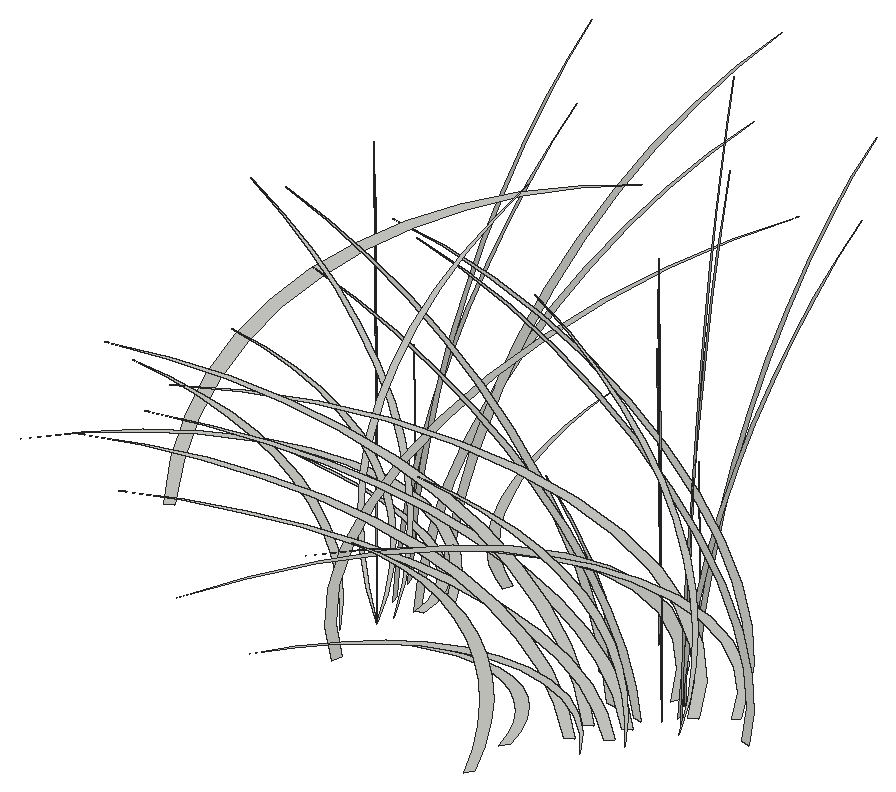
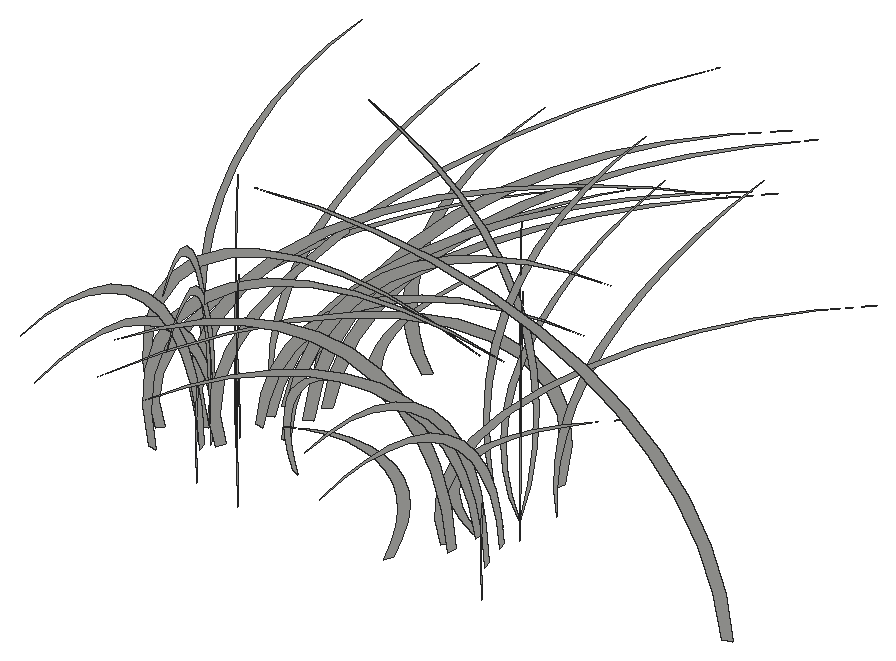
# SketchUp Ruby script. Lengths in inches.
U = 1.inch
M = Sketchup.active_model
def pt(a) = Geom::Point3d.new(a.map { |v| v * U })
def face(e, loops, mat)
  f = e.add_face(loops[0].map { |a| pt(a) })
  loops[1..].each { |l| e.add_face(l.map { |a| pt(a) }).erase! }
  f.material = f.back_material = mat if mat
  f
end
# faces: each face lists its corners as indices into pts; further lists are holes
def faces(e, pts, list, mat = nil) = list.each { |f| face(e, (f[0].is_a?(Array) ? f : [f]).map { |l| l.map { |i| pts[i] } }, mat) }
# xy, xz, yz: faces in a plane at the given z, y or x. An outline is a flat list of corners, or four numbers for a rectangle; further outlines are holes
def ring(l) = l.size == 4 ? [[l[0], l[1]], [l[2], l[1]], [l[2], l[3]], [l[0], l[3]]] : l.each_slice(2).to_a
def flat(e, list, mat, &to3) = list.each { |f| face(e, (f[0].is_a?(Array) ? f : [f]).map { |l| ring(l).map { |u, v| to3.(u, v) } }, mat) }
def xy(e, z, list, mat = nil) = flat(e, list, mat) { |x, y| [x, y, z] }
def xz(e, y, list, mat = nil) = flat(e, list, mat) { |x, z| [x, y, z] }
def yz(e, x, list, mat = nil) = flat(e, list, mat) { |y, z| [x, y, z] }
def lines(e, pts, list) = list.each { |a, b| e.add_line(pt(pts[a]), pt(pts[b])) }
# prism: a flat outline (further loops are holes) pulled along v
def prism(e, loops, v, mat = nil)
  f = face(e, loops, mat); d = Geom::Vector3d.new(v.map { |x| x * U })
  f.pushpull(f.normal.samedirection?(d) ? d.length : -d.length)
end
def box(e, o, s, mat = nil) = prism(e, [[o, [o[0] + s[0], o[1], o[2]], [o[0] + s[0], o[1] + s[1], o[2]], [o[0], o[1] + s[1], o[2]]]], [0, 0, s[2]], mat)
def at(x, y, z, deg = 0) = Geom::Transformation.translation(pt([x, y, z])) * Geom::Transformation.rotation(ORIGIN, Z_AXIS, deg.degrees)
def axes(o, x, y, z) = Geom::Transformation.new([*x, 0, *y, 0, *z, 0, *pt(o).to_a, 1])
def part(name) = M.definitions.add(name)
# library, detail: a bought-in or finely detailed component or shape, given as its bounding box
def library(name, o, s) = part(name).tap { |d| box(d.entities, o, s) }
def detail(e, o, s) = box(e.add_group.entities, o, s)
def put(e, d, t, mat = nil) = e.add_instance(d, t).tap { |i| i.material = mat if mat }
def group(e, t, mat = nil) = e.add_group.tap { |g| g.transformation = t; g.material = mat if mat }.entities
root = M.entities
g1 = group(root,at(387.49,274.53,0))
p = [[-0.5,-0.57,0],[-0.22,-0.25,0],[0,0,1.46],[-0.09,-0.1,2.93],[-0.49,-0.56,4.375],[-1.19,-1.35,5.75],
  [-2.17,-2.47,7.03],[-3.41,-3.89,8.18],[-4.88,-5.56,9.17],[-6.54,-7.45,9.98],[-8.36,-9.51,10.58],[-10.27,-11.69,10.97],
  [-12.24,-13.9375,11.125],[-14.23,-16.19,11.05],[-12.28,-13.98,11.0625],[-10.36,-11.79,10.86],[-8.5,-9.67,10.44],[-6.74,-7.67,9.82],
  [-5.13,-5.84,9.01],[-3.71,-4.22,8.02],[-2.51,-2.85,6.89],[-1.54,-1.76,5.64],[-0.85,-0.97,4.29],[-0.44,-0.5,2.88],
  [-0.32,-0.37,1.4375]]
faces(g1,p,[[0,1,2,3,4,5,6,7,8,9,10,11,12,13,14,15,16,17,18,19,20,21,22,23,24]])
g2 = group(root,at(384.38,274.21,0))
p = [[-6.07,19.87,18.05],[-6.99,22.87,18.53],[-6.1,19.96,17.95],[-5.25,17.16,17.15],[-4.43,14.49,16.14],[-3.66,11.97,14.93],
  [-2.95,9.65,13.53],[-2.31,7.54,11.96],[-1.73,5.67,10.23],[-1.24,4.06,8.37],[-0.83,2.72,6.39],[-0.51,1.68,4.32],
  [-0.29,0.94,2.18],[-0.16,0.52,0],[0,0,0],[-0.11,0.35,2.23],[-0.32,1.04,4.43],[-0.63,2.07,6.55],
  [-1.04,3.41,8.57],[-1.55,5.05,10.47],[-2.13,6.98,12.22],[-2.8,9.16,13.8],[-3.54,11.58,15.1875],[-4.34,14.1875,16.37],
  [-5.1875,16.96,17.33]]
faces(g2,p,[[0,1,2,3,4,5,6,7,8,9,10,11,12,13,14,15,16,17,18,19,20,21,22,23,24]])
g3 = group(root,at(383.32,276.15,0))
p = [[-4.56,5.55,7.88],[-3.72,4.53,7.38],[-2.97,3.62,6.83],[-2.31,2.81,6.24],[-1.73,2.11,5.62],[-1.26,1.54,4.96],
  [-0.89,1.09,4.27],[-0.63,0.76,3.57],[-0.47,0.58,2.86],[-0.43,0.52,2.13],[-0.49,0.6,1.41],[-0.67,0.81,0.7],
  [-0.95,1.16,0],[-0.59,0.71,0],[-0.27,0.33,0.71],[-0.07,0.09,1.43],[0,0,2.17],[-0.05,0.0625,2.9],
  [-0.22,0.27,3.63],[-0.52,0.63,4.34],[-0.93,1.13,5.03],[-1.45,1.77,5.69],[-2.09,2.54,6.3125],[-2.82,3.43,6.89],
  [-3.65,4.44,7.41]]
faces(g3,p,[[0,1,2,3,4,5,6,7,8,9,10,11,12,13,14,15,16,17,18,19,20,21,22,23,24]])
g4 = group(root,at(384.6,271.54,0))
p = [[-6.74,8.21,19.61],[-5.67,6.9,18.16],[-4.68,5.7,16.67],[-3.78,4.6,15.125],[-2.98,3.62,13.55],[-2.27,2.76,11.93],
  [-1.65,2.01,10.28],[-1.14,1.39,8.61],[-0.72,0.88,6.91],[-0.41,0.5,5.2],[-0.2,0.24,3.47],[-0.09,0.11,1.74],
  [-0.09,0.11,0],[0,0,1.74],[-0.03,0.04,3.49],[-0.1875,0.23,5.23],[-0.46,0.56,6.96],[-0.85,1.04,8.67],
  [-1.36,1.66,10.36],[-1.98,2.42,12.01],[-2.72,3.3125,13.63],[-3.57,4.35,15.21],[-4.52,5.51,16.73],[-5.58,6.8,18.2]]
faces(g4,p,[[0,1,2,3,4,5,6,7,8,9,10,11,12,13,14,15,16,17,18,19,20,21,22,23]])
g5 = group(root,at(384.6,271.54,0))
p = [[-6.74,8.21,19.61],[-5.67,6.9,18.16],[-4.68,5.7,16.67],[-3.78,4.6,15.125],[-2.98,3.62,13.55],[-2.27,2.76,11.93],
  [-1.65,2.01,10.28],[-1.14,1.39,8.61],[-0.72,0.88,6.91],[-0.41,0.5,5.2],[-0.2,0.24,3.47],[-0.09,0.11,1.74],
  [-0.09,0.11,0],[0,0,1.74],[-0.03,0.04,3.49],[-0.1875,0.23,5.23],[-0.46,0.56,6.96],[-0.85,1.04,8.67],
  [-1.36,1.66,10.36],[-1.98,2.42,12.01],[-2.72,3.3125,13.63],[-3.57,4.35,15.21],[-4.52,5.51,16.73],[-5.58,6.8,18.2]]
faces(g5,p,[[0,1,2,3,4,5,6,7,8,9,10,11,12,13,14,15,16,17,18,19,20,21,22,23]])
g6 = group(root,at(370.36,272.98,0.02))
p = [[19.18,7.98,20.75],[22.08,9.1875,21.3],[19.27,8.02,20.63],[16.57,6.9,19.72],[13.98,5.82,18.55],[11.56,4.8125,17.16],
  [9.32,3.88,15.55],[7.28,3.03,13.74],[5.47,2.28,11.76],[3.92,1.63,9.62],[2.63,1.09,7.35],[1.625,0.68,4.97],
  [0.91,0.38,2.51],[0.5,0.21,0],[0,0,0],[0.34,0.14,2.57],[1.01,0.42,5.09],[1.99,0.83,7.53],
  [3.29,1.37,9.85],[4.88,2.03,12.03],[6.74,2.81,14.04],[8.85,3.68,15.86],[11.18,4.65,17.46],[13.7,5.7,18.82],
  [16.375,6.82,19.92]]
faces(g6,p,[[0,1,2,3,4,5,6,7,8,9,10,11,12,13,14,15,16,17,18,19,20,21,22,23,24]])
g7 = group(root,at(384.94,272.36,0))
p = [[-6.07,19.87,14.56],[-6.99,22.87,14.94],[-6.1,19.96,14.48],[-5.25,17.16,13.83],[-4.43,14.49,13.02],[-3.66,11.97,12.04],
  [-2.95,9.65,10.91],[-2.31,7.54,9.64],[-1.73,5.67,8.25],[-1.24,4.06,6.75],[-0.83,2.72,5.15],[-0.51,1.68,3.49],
  [-0.29,0.94,1.76],[-0.16,0.52,0],[0,0,0],[-0.11,0.35,1.8],[-0.32,1.04,3.57],[-0.63,2.07,5.28],
  [-1.04,3.41,6.91],[-1.55,5.05,8.44],[-2.13,6.98,9.85],[-2.8,9.16,11.13],[-3.54,11.58,12.25],[-4.34,14.1875,13.2],
  [-5.1875,16.96,13.97]]
faces(g7,p,[[0,1,2,3,4,5,6,7,8,9,10,11,12,13,14,15,16,17,18,19,20,21,22,23,24]])
g8 = group(root,at(384.75,268.79,0))
p = [[-5.83,-8.875,16.67],[-4.9,-7.46,15.44],[-4.05,-6.16,14.17],[-3.27,-4.98,12.86],[-2.58,-3.92,11.51],[-1.96,-2.98,10.14],
  [-1.43,-2.18,8.74],[-0.99,-1.5,7.31],[-0.63,-0.95,5.87],[-0.36,-0.54,4.42],[-0.17,-0.26,2.95],[-0.08,-0.12,1.48],
  [-0.08,-0.12,0],[0,0,1.48],[-0.03,-0.04,2.97],[-0.16,-0.24,4.45],[-0.4,-0.6,5.92],[-0.74,-1.12,7.37],
  [-1.18,-1.79,8.81],[-1.72,-2.61,10.21],[-2.36,-3.58,11.59],[-3.09,-4.7,12.93],[-3.92,-5.96,14.22],[-4.83,-7.35,15.47]]
faces(g8,p,[[0,1,2,3,4,5,6,7,8,9,10,11,12,13,14,15,16,17,18,19,20,21,22,23]])
g9 = group(root,at(386.86,271.52,0))
p = [[-0.89,-0.32,0],[-0.4,-0.14,1.97],[-0.1,-0.04,3.96],[0,0,5.95],[-0.1,-0.03,7.95],[-0.39,-0.14,9.9375],
  [-0.89,-0.3125,11.91],[-1.57,-0.56,13.85],[-2.45,-0.87,15.76],[-3.52,-1.25,17.63],[-4.77,-1.6875,19.44],[-6.19,-2.19,21.2],
  [-7.79,-2.76,22.89],[-6.29,-2.23,21.17],[-4.94,-1.75,19.4],[-3.76,-1.33,17.58],[-2.74,-0.97,15.71],[-1.89,-0.67,13.8],
  [-1.22,-0.43,11.86],[-0.72,-0.25,9.9],[-0.4,-0.14,7.93],[-0.25,-0.09,5.94],[-0.29,-0.1,3.95],[-0.5,-0.18,1.97]]
faces(g9,p,[[0,1,2,3,4,5,6,7,8,9,10,11,12,13,14,15,16,17,18,19,20,21,22,23]])
g10 = group(root,at(387.96,272.875,0))
p = [[-9.01,-2.98,7.88],[-7.3,-2.41,7.38],[-5.75,-1.9,6.83],[-4.38,-1.45,6.24],[-3.2,-1.06,5.62],[-2.23,-0.74,4.96],
  [-1.47,-0.49,4.27],[-0.92,-0.31,3.57],[-0.61,-0.2,2.86],[-0.51,-0.17,2.13],[-0.65,-0.21,1.41],[-1.01,-0.33,0.7],
  [-1.6,-0.53,0],[-1.21,-0.4,0],[-0.54,-0.18,0.69],[-0.12,-0.04,1.4],[0.06,0.02,2.13],[-0.02,-0.01,2.85],
  [-0.35,-0.11,3.58],[-0.92,-0.3,4.29],[-1.73,-0.57,4.98],[-2.78,-0.92,5.64],[-4.05,-1.34,6.27],[-5.52,-1.82,6.86],
  [-7.18,-2.375,7.4]]
faces(g10,p,[[0,1,2,3,4,5,6,7,8,9,10,11,12,13,14,15,16,17,18,19,20,21,22,23,24]])
g11 = group(root,at(386.29,269.49,0))
p = [[-0.6,0.73,0],[-0.27,0.33,1.77],[-0.07,0.08,3.57],[0,0,5.36],[-0.07,0.08,7.16],[-0.27,0.32,8.95],
  [-0.6,0.73,10.73],[-1.06,1.29,12.48],[-1.65,2.01,14.2],[-2.37,2.88,15.88],[-3.21,3.91,17.52],[-4.17,5.08,19.1],
  [-5.25,6.39,20.625],[-4.23,5.15,19.08],[-3.33,4.05,17.48],[-2.53,3.08,15.83],[-1.84,2.25,14.15],[-1.27,1.55,12.43],
  [-0.82,1,10.6875],[-0.48,0.59,8.92],[-0.27,0.32,7.14],[-0.17,0.21,5.35],[-0.19,0.24,3.5625],[-0.34,0.41,1.78]]
faces(g11,p,[[0,1,2,3,4,5,6,7,8,9,10,11,12,13,14,15,16,17,18,19,20,21,22,23]])
g12 = group(root,at(386.21,271.01,0))
p = [[-0.52,-0.79,0],[-0.23,-0.35,1.51],[-0.06,-0.09,3.03],[0,0,4.56],[-0.06,-0.09,6.09],[-0.23,-0.35,7.61],
  [-0.52,-0.79,9.12],[-0.92,-1.39,10.61],[-1.43,-2.17,12.07],[-2.05,-3.12,13.5],[-2.78,-4.23,14.89],[-3.61,-5.49,16.24],
  [-4.54,-6.91,17.53],[-3.66,-5.57,16.21],[-2.88,-4.38,14.86],[-2.1875,-3.33,13.46],[-1.6,-2.43,12.03],[-1.1,-1.68,10.57],
  [-0.71,-1.08,9.08],[-0.42,-0.64,7.58],[-0.23,-0.35,6.07],[-0.15,-0.22,4.55],[-0.17,-0.25,3.03],[-0.29,-0.44,1.51]]
faces(g12,p,[[0,1,2,3,4,5,6,7,8,9,10,11,12,13,14,15,16,17,18,19,20,21,22,23]])
g13 = group(root,at(386.3125,272.24,0))
p = [[1.63,20.71,16.73],[1.875,23.84,17.17],[1.64,20.8125,16.64],[1.41,17.89,15.9],[1.1875,15.1,14.96],[0.98,12.48,13.84],
  [0.79,10.06,12.54],[0.62,7.86,11.08],[0.47,5.91,9.48],[0.33,4.23,7.76],[0.22,2.84,5.92],[0.14,1.75,4.01],
  [0.08,0.98,2.02],[0.04,0.54,0],[0,0,0],[0.03,0.36,2.07],[0.09,1.09,4.1],[0.17,2.15,6.07],
  [0.28,3.55,7.94],[0.41,5.27,9.7],[0.57,7.28,11.33],[0.75,9.55,12.79],[0.95,12.07,14.08],[1.16,14.79,15.17],
  [1.39,17.68,16.0625]]
faces(g13,p,[[0,1,2,3,4,5,6,7,8,9,10,11,12,13,14,15,16,17,18,19,20,21,22,23,24]])
g14 = group(root,at(386.47,274.17,0))
p = [[1.63,20.71,20.75],[1.875,23.84,21.3],[1.64,20.8125,20.63],[1.41,17.89,19.72],[1.1875,15.1,18.55],[0.98,12.48,17.16],
  [0.79,10.06,15.55],[0.62,7.86,13.74],[0.47,5.91,11.76],[0.33,4.23,9.62],[0.22,2.84,7.35],[0.14,1.75,4.97],
  [0.08,0.98,2.51],[0.04,0.54,0],[0,0,0],[0.03,0.36,2.57],[0.09,1.09,5.09],[0.17,2.15,7.53],
  [0.28,3.55,9.85],[0.41,5.27,12.03],[0.57,7.28,14.04],[0.75,9.55,15.86],[0.95,12.07,17.46],[1.16,14.79,18.82],
  [1.39,17.68,19.92]]
faces(g14,p,[[0,1,2,3,4,5,6,7,8,9,10,11,12,13,14,15,16,17,18,19,20,21,22,23,24]])
g15 = group(root,at(399.7,270.96,0))
p = [[-20.46,3.64,18.05],[-23.54,4.19,18.53],[-20.55,3.66,17.95],[-17.67,3.15,17.15],[-14.91,2.66,16.14],[-12.33,2.2,14.93],
  [-9.93,1.77,13.53],[-7.76,1.38,11.96],[-5.84,1.04,10.23],[-4.18,0.74,8.37],[-2.8,0.5,6.39],[-1.73,0.31,4.32],
  [-0.97,0.17,2.18],[-0.53,0.09,0],[0,0,0],[-0.36,0.0625,2.23],[-1.07,0.19,4.43],[-2.125,0.38,6.55],
  [-3.51,0.625,8.57],[-5.2,0.93,10.47],[-7.1875,1.28,12.22],[-9.43,1.68,13.8],[-11.92,2.125,15.1875],[-14.61,2.6,16.37],
  [-17.46,3.11,17.33]]
faces(g15,p,[[0,1,2,3,4,5,6,7,8,9,10,11,12,13,14,15,16,17,18,19,20,21,22,23,24]])
g16 = group(root,at(385.02,269.55,0))
p = [[0.67,0.67,0],[0.3,0.3,2.04],[0.08,0.08,4.1],[0,0,6.17],[0.07,0.07,8.23],[0.3,0.3,10.29],
  [0.66,0.66,12.33],[1.18,1.18,14.34],[1.84,1.84,16.32],[2.64,2.64,18.26],[3.58,3.58,20.14],[4.65,4.65,21.96],
  [5.84,5.84,23.71],[4.72,4.72,21.93],[3.71,3.71,20.09],[2.82,2.82,18.2],[2.05,2.05,16.26],[1.42,1.42,14.29],
  [0.91,0.91,12.29],[0.54,0.54,10.26],[0.3,0.3,8.21],[0.1875,0.1875,6.15],[0.22,0.22,4.09],[0.375,0.375,2.04]]
faces(g16,p,[[0,1,2,3,4,5,6,7,8,9,10,11,12,13,14,15,16,17,18,19,20,21,22,23]])
g17 = group(root,at(388.01,275.77,0))
p = [[2.34,6.79,9.0625],[1.91,5.55,8.49],[1.52,4.43,7.85],[1.18,3.44,7.18],[0.89,2.58,6.45],[0.65,1.88,5.7],
  [0.46,1.33,4.91],[0.32,0.93,4.1],[0.24,0.7,3.28],[0.22,0.64,2.45],[0.25,0.74,1.625],[0.34,1,0.8],
  [0.49,1.42,0],[0.3,0.875,0],[0.14,0.4,0.81],[0.04,0.11,1.65],[0,0,2.49],[0.03,0.07,3.34],
  [0.11,0.33,4.17],[0.27,0.77,4.99],[0.48,1.38,5.79],[0.75,2.17,6.54],[1.07,3.11,7.26],[1.45,4.2,7.92],
  [1.87,5.43,8.52]]
faces(g17,p,[[0,1,2,3,4,5,6,7,8,9,10,11,12,13,14,15,16,17,18,19,20,21,22,23,24]])
g18 = group(root,at(400.09,268.86,0))
p = [[-18.45,-9.5625,18.05],[-21.23,-11,18.53],[-18.53,-9.61,17.95],[-15.93,-8.26,17.15],[-13.45,-6.97,16.14],[-11.12,-5.76,14.93],
  [-8.96,-4.64,13.53],[-7,-3.63,11.96],[-5.26,-2.73,10.23],[-3.77,-1.95,8.37],[-2.53,-1.3125,6.39],[-1.5625,-0.81,4.32],
  [-0.875,-0.45,2.18],[-0.48,-0.25,0],[0,0,0],[-0.32,-0.17,2.23],[-0.97,-0.5,4.43],[-1.92,-0.99,6.55],
  [-3.16,-1.64,8.57],[-4.69,-2.43,10.47],[-6.48,-3.36,12.22],[-8.51,-4.41,13.8],[-10.75,-5.57,15.1875],[-13.17,-6.83,16.37],
  [-15.75,-8.16,17.33]]
faces(g18,p,[[0,1,2,3,4,5,6,7,8,9,10,11,12,13,14,15,16,17,18,19,20,21,22,23,24]])
g19 = group(root,at(400.09,268.86,0))
p = [[-18.45,-9.5625,18.05],[-21.23,-11,18.53],[-18.53,-9.61,17.95],[-15.93,-8.26,17.15],[-13.45,-6.97,16.14],[-11.12,-5.76,14.93],
  [-8.96,-4.64,13.53],[-7,-3.63,11.96],[-5.26,-2.73,10.23],[-3.77,-1.95,8.37],[-2.53,-1.3125,6.39],[-1.5625,-0.81,4.32],
  [-0.875,-0.45,2.18],[-0.48,-0.25,0],[0,0,0],[-0.32,-0.17,2.23],[-0.97,-0.5,4.43],[-1.92,-0.99,6.55],
  [-3.16,-1.64,8.57],[-4.69,-2.43,10.47],[-6.48,-3.36,12.22],[-8.51,-4.41,13.8],[-10.75,-5.57,15.1875],[-13.17,-6.83,16.37],
  [-15.75,-8.16,17.33]]
faces(g19,p,[[0,1,2,3,4,5,6,7,8,9,10,11,12,13,14,15,16,17,18,19,20,21,22,23,24]])
g20 = group(root,at(401.6,270.62,0))
p = [[-20.46,3.64,14.56],[-23.54,4.19,14.94],[-20.55,3.66,14.48],[-17.67,3.15,13.83],[-14.91,2.66,13.02],[-12.33,2.2,12.04],
  [-9.93,1.77,10.91],[-7.76,1.38,9.64],[-5.84,1.04,8.25],[-4.18,0.74,6.75],[-2.8,0.5,5.15],[-1.73,0.31,3.49],
  [-0.97,0.17,1.76],[-0.53,0.09,0],[0,0,0],[-0.36,0.0625,1.8],[-1.07,0.19,3.57],[-2.125,0.38,5.28],
  [-3.51,0.625,6.91],[-5.2,0.93,8.44],[-7.1875,1.28,9.85],[-9.43,1.68,11.13],[-11.92,2.125,12.25],[-14.61,2.6,13.2],
  [-17.46,3.11,13.97]]
faces(g20,p,[[0,1,2,3,4,5,6,7,8,9,10,11,12,13,14,15,16,17,18,19,20,21,22,23,24]])
g21 = group(root,at(386.16,265.61,0))
p = [[0.26,0.96,0],[0.11,0.43,0],[0,0,2.01],[0.05,0.17,4.04],[0.25,0.9375,6.02],[0.62,2.28,7.92],
  [1.125,4.16,9.68],[1.76,6.54,11.26],[2.52,9.35,12.62],[3.38,12.53,13.73],[4.32,16,14.5625],[5.31,19.67,15.09],
  [6.33,23.45,15.31],[7.35,27.24,15.2],[6.35,23.52,15.22],[5.35,19.83,14.94],[4.39,16.27,14.37],[3.48,12.91,13.51],
  [2.65,9.83,12.39],[1.92,7.11,11.04],[1.29,4.8,9.48],[0.8,2.96,7.75],[0.44,1.63,5.9],[0.23,0.84,3.96],
  [0.17,0.62,1.98]]
faces(g21,p,[[0,1,2,3,4,5,6,7,8,9,10,11,12,13,14,15,16,17,18,19,20,21,22,23,24]])
g22 = group(root,at(400.14,267.37,0))
p = [[-17.17,-11.7,15.34],[-19.76,-13.47,15.75],[-17.25,-11.76,15.26],[-14.83,-10.11,14.58],[-12.52,-8.53,13.72],[-10.35,-7.05,12.69],
  [-8.34,-5.68,11.5],[-6.52,-4.44,10.16],[-4.9,-3.34,8.7],[-3.51,-2.39,7.11],[-2.35,-1.6,5.43],[-1.45,-0.99,3.67],
  [-0.82,-0.56,1.86],[-0.45,-0.3,0],[0,0,0],[-0.3,-0.21,1.9],[-0.9,-0.61,3.76],[-1.78,-1.22,5.57],
  [-2.95,-2.01,7.28],[-4.37,-2.98,8.9],[-6.03,-4.11,10.39],[-7.92,-5.4,11.73],[-10,-6.82,12.91],[-12.26,-8.36,13.91],
  [-14.66,-9.99,14.73]]
faces(g22,p,[[0,1,2,3,4,5,6,7,8,9,10,11,12,13,14,15,16,17,18,19,20,21,22,23,24]])
g23 = group(root,at(401.81,269.75,0))
p = [[-18.45,-9.5625,14.56],[-21.23,-11,14.94],[-18.53,-9.61,14.48],[-15.93,-8.26,13.83],[-13.45,-6.97,13.02],[-11.12,-5.76,12.04],
  [-8.96,-4.64,10.91],[-7,-3.63,9.64],[-5.26,-2.73,8.25],[-3.77,-1.95,6.75],[-2.53,-1.3125,5.15],[-1.5625,-0.81,3.49],
  [-0.875,-0.45,1.76],[-0.48,-0.25,0],[0,0,0],[-0.32,-0.17,1.8],[-0.97,-0.5,3.57],[-1.92,-0.99,5.28],
  [-3.16,-1.64,6.91],[-4.69,-2.43,8.44],[-6.48,-3.36,9.85],[-8.51,-4.41,11.13],[-10.75,-5.57,12.25],[-13.17,-6.83,13.2],
  [-15.75,-8.16,13.97]]
faces(g23,p,[[0,1,2,3,4,5,6,7,8,9,10,11,12,13,14,15,16,17,18,19,20,21,22,23,24]])
g24 = group(root,at(401.81,269.75,0))
p = [[-18.45,-9.5625,14.56],[-21.23,-11,14.94],[-18.53,-9.61,14.48],[-15.93,-8.26,13.83],[-13.45,-6.97,13.02],[-11.12,-5.76,12.04],
  [-8.96,-4.64,10.91],[-7,-3.63,9.64],[-5.26,-2.73,8.25],[-3.77,-1.95,6.75],[-2.53,-1.3125,5.15],[-1.5625,-0.81,3.49],
  [-0.875,-0.45,1.76],[-0.48,-0.25,0],[0,0,0],[-0.32,-0.17,1.8],[-0.97,-0.5,3.57],[-1.92,-0.99,5.28],
  [-3.16,-1.64,6.91],[-4.69,-2.43,8.44],[-6.48,-3.36,9.85],[-8.51,-4.41,11.13],[-10.75,-5.57,12.25],[-13.17,-6.83,13.2],
  [-15.75,-8.16,13.97]]
faces(g24,p,[[0,1,2,3,4,5,6,7,8,9,10,11,12,13,14,15,16,17,18,19,20,21,22,23,24]])
g25 = group(root,at(404.67,275.47,0))
p = [[-0.91,0.16,0],[-0.4,0.07,0],[0,0,2.0625],[-0.16,0.03,4.13],[-0.89,0.16,6.16],[-2.17,0.39,8.1],
  [-3.95,0.7,9.91],[-6.21,1.11,11.52],[-8.88,1.58,12.92],[-11.91,2.12,14.05],[-15.2,2.71,14.9],[-18.68,3.33,15.45],
  [-22.27,3.97,15.67],[-25.88,4.61,15.5625],[-22.34,3.98,15.58],[-18.84,3.36,15.29],[-15.45,2.75,14.71],[-12.26,2.18,13.83],
  [-9.34,1.66,12.68],[-6.75,1.2,11.3],[-4.56,0.8125,9.7],[-2.81,0.5,7.9375],[-1.55,0.28,6.04],[-0.8,0.14,4.05],
  [-0.59,0.1,2.02]]
faces(g25,p,[[0,1,2,3,4,5,6,7,8,9,10,11,12,13,14,15,16,17,18,19,20,21,22,23,24]])
g26 = group(root,at(404.67,275.47,0))
p = [[-0.91,0.16,0],[-0.4,0.07,0],[0,0,2.0625],[-0.16,0.03,4.13],[-0.89,0.16,6.16],[-2.17,0.39,8.1],
  [-3.95,0.7,9.91],[-6.21,1.11,11.52],[-8.88,1.58,12.92],[-11.91,2.12,14.05],[-15.2,2.71,14.9],[-18.68,3.33,15.45],
  [-22.27,3.97,15.67],[-25.88,4.61,15.5625],[-22.34,3.98,15.58],[-18.84,3.36,15.29],[-15.45,2.75,14.71],[-12.26,2.18,13.83],
  [-9.34,1.66,12.68],[-6.75,1.2,11.3],[-4.56,0.8125,9.7],[-2.81,0.5,7.9375],[-1.55,0.28,6.04],[-0.8,0.14,4.05],
  [-0.59,0.1,2.02]]
faces(g26,p,[[0,1,2,3,4,5,6,7,8,9,10,11,12,13,14,15,16,17,18,19,20,21,22,23,24]])
g27 = group(root,at(401.73,268.46,0))
p = [[-17.17,-11.7,12.375],[-19.76,-13.47,12.7],[-17.25,-11.76,12.31],[-14.83,-10.11,11.76],[-12.52,-8.53,11.07],[-10.35,-7.05,10.23],
  [-8.34,-5.68,9.27],[-6.52,-4.44,8.2],[-4.9,-3.34,7.01],[-3.51,-2.39,5.74],[-2.35,-1.6,4.38],[-1.45,-0.99,2.96],
  [-0.82,-0.56,1.5],[-0.45,-0.3,0],[0,0,0],[-0.3,-0.21,1.53],[-0.9,-0.61,3.03],[-1.78,-1.22,4.49],
  [-2.95,-2.01,5.875],[-4.37,-2.98,7.18],[-6.03,-4.11,8.375],[-7.92,-5.4,9.46],[-10,-6.82,10.41],[-12.26,-8.36,11.22],
  [-14.66,-9.99,11.88]]
faces(g27,p,[[0,1,2,3,4,5,6,7,8,9,10,11,12,13,14,15,16,17,18,19,20,21,22,23,24]])
g28 = group(root,at(403.93,272.77,0))
p = [[-0.82,-0.43,0],[-0.36,-0.1875,0],[0,0,2.0625],[-0.15,-0.08,4.13],[-0.8,-0.42,6.16],[-1.95,-1.01,8.1],
  [-3.57,-1.85,9.91],[-5.6,-2.9,11.52],[-8.01,-4.15,12.92],[-10.74,-5.57,14.05],[-13.71,-7.1,14.9],[-16.85,-8.73,15.45],
  [-20.09,-10.41,15.67],[-23.34,-12.1,15.5625],[-20.15,-10.44,15.58],[-16.99,-8.81,15.29],[-13.9375,-7.22,14.71],[-11.06,-5.73,13.83],
  [-8.42,-4.37,12.68],[-6.09,-3.16,11.3],[-4.11,-2.13,9.7],[-2.53,-1.3125,7.9375],[-1.4,-0.72,6.04],[-0.72,-0.375,4.05],
  [-0.53,-0.27,2.02]]
faces(g28,p,[[0,1,2,3,4,5,6,7,8,9,10,11,12,13,14,15,16,17,18,19,20,21,22,23,24]])
g29 = group(root,at(407.53,271.91,0))
p = [[-0.95,0.28,0],[-0.42,0.125,0],[0,0,2.01],[-0.17,0.05,4.04],[-0.93,0.27,6.02],[-2.27,0.66,7.92],
  [-4.14,1.21,9.68],[-6.5,1.9,11.26],[-9.3,2.72,12.62],[-12.46,3.64,13.73],[-15.91,4.65,14.5625],[-19.55,5.72,15.09],
  [-23.3125,6.82,15.31],[-27.08,7.92,15.2],[-23.38,6.84,15.22],[-19.72,5.77,14.94],[-16.17,4.73,14.37],[-12.83,3.75,13.51],
  [-9.77,2.86,12.39],[-7.0625,2.07,11.04],[-4.77,1.39,9.48],[-2.94,0.86,7.75],[-1.62,0.47,5.9],[-0.84,0.25,3.96],
  [-0.61,0.18,1.98]]
faces(g29,p,[[0,1,2,3,4,5,6,7,8,9,10,11,12,13,14,15,16,17,18,19,20,21,22,23,24]])
g30 = group(root,at(398.26,272.65,0))
p = [[-6.53,2.99,7.88],[-5.33,2.44,7.38],[-4.26,1.95,6.83],[-3.3,1.51,6.24],[-2.48,1.14,5.62],[-1.81,0.83,4.96],
  [-1.28,0.58,4.27],[-0.9,0.41,3.57],[-0.68,0.31,2.86],[-0.61,0.28,2.13],[-0.71,0.32,1.41],[-0.96,0.4375,0.7],
  [-1.37,0.625,0],[-0.84,0.38,0],[-0.39,0.18,0.71],[-0.11,0.05,1.43],[0,0,2.17],[-0.07,0.03,2.9],
  [-0.32,0.15,3.63],[-0.74,0.34,4.34],[-1.33,0.61,5.03],[-2.08,0.95,5.69],[-2.99,1.37,6.3125],[-4.04,1.85,6.89],
  [-5.22,2.39,7.41]]
faces(g30,p,[[0,1,2,3,4,5,6,7,8,9,10,11,12,13,14,15,16,17,18,19,20,21,22,23,24]])
g31 = group(root,at(401.02,272.88,0))
p = [[-10.66,12.98,9.9],[-9.23,11.23,9.83],[-7.82,9.52,9.59],[-6.46,7.86,9.18],[-5.18,6.3,8.61],[-3.99,4.86,7.88],
  [-2.93,3.57,7.02],[-2.02,2.46,6.03],[-1.27,1.54,4.95],[-0.6875,0.84,3.78],[-0.29,0.36,2.55],[-0.1,0.12,1.28],
  [-0.09,0.12,0],[0,0,1.3],[-0.125,0.15,2.61],[-0.47,0.57,3.875],[-1.02,1.24,5.09],[-1.77,2.15,6.21],
  [-2.69,3.28,7.22],[-3.78,4.6,8.1],[-5,6.09,8.82],[-6.33,7.71,9.37],[-7.74,9.43,9.74],[-9.2,11.19,9.92]]
faces(g31,p,[[0,1,2,3,4,5,6,7,8,9,10,11,12,13,14,15,16,17,18,19,20,21,22,23]])
g32 = group(root,at(402.28,273.16,0))
p = [[-11.32,17.43,20.75],[-13.02,20.05,21.3],[-11.37,17.51,20.63],[-9.77,15.05,19.72],[-8.25,12.7,18.55],[-6.82,10.5,17.16],
  [-5.5,8.46,15.55],[-4.29,6.61,13.74],[-3.23,4.97,11.76],[-2.3125,3.56,9.62],[-1.55,2.39,7.35],[-0.96,1.47,4.97],
  [-0.54,0.83,2.51],[-0.29,0.45,0],[0,0,0],[-0.2,0.31,2.57],[-0.59,0.91,5.09],[-1.18,1.8125,7.53],
  [-1.94,2.99,9.85],[-2.88,4.43,12.03],[-3.98,6.12,14.04],[-5.22,8.04,15.86],[-6.59,10.15,17.46],[-8.08,12.44,18.82],
  [-9.66,14.88,19.92]]
faces(g32,p,[[0,1,2,3,4,5,6,7,8,9,10,11,12,13,14,15,16,17,18,19,20,21,22,23,24]])
g33 = group(root,at(398.15,276.375,0))
p = [[-4.56,5.55,16.02],[-3.72,4.53,15.01],[-2.97,3.62,13.89],[-2.31,2.81,12.69],[-1.73,2.11,11.42],[-1.26,1.54,10.08],
  [-0.89,1.09,8.6875],[-0.63,0.76,7.26],[-0.47,0.58,5.8],[-0.43,0.52,4.34],[-0.49,0.6,2.87],[-0.67,0.81,1.42],
  [-0.95,1.16,0],[-0.59,0.71,0],[-0.27,0.33,1.44],[-0.07,0.09,2.92],[0,0,4.41],[-0.05,0.0625,5.9],
  [-0.22,0.27,7.38],[-0.52,0.63,8.83],[-0.93,1.13,10.23],[-1.45,1.77,11.57],[-2.09,2.54,12.83],[-2.82,3.43,14.01],
  [-3.65,4.44,15.07]]
faces(g33,p,[[0,1,2,3,4,5,6,7,8,9,10,11,12,13,14,15,16,17,18,19,20,21,22,23,24]])
g34 = group(root,at(398.15,276.375,0))
p = [[-4.56,5.55,16.02],[-3.72,4.53,15.01],[-2.97,3.62,13.89],[-2.31,2.81,12.69],[-1.73,2.11,11.42],[-1.26,1.54,10.08],
  [-0.89,1.09,8.6875],[-0.63,0.76,7.26],[-0.47,0.58,5.8],[-0.43,0.52,4.34],[-0.49,0.6,2.87],[-0.67,0.81,1.42],
  [-0.95,1.16,0],[-0.59,0.71,0],[-0.27,0.33,1.44],[-0.07,0.09,2.92],[0,0,4.41],[-0.05,0.0625,5.9],
  [-0.22,0.27,7.38],[-0.52,0.63,8.83],[-0.93,1.13,10.23],[-1.45,1.77,11.57],[-2.09,2.54,12.83],[-2.82,3.43,14.01],
  [-3.65,4.44,15.07]]
faces(g34,p,[[0,1,2,3,4,5,6,7,8,9,10,11,12,13,14,15,16,17,18,19,20,21,22,23,24]])
g35 = group(root,at(401.85,273.96,0))
p = [[-0.37,-0.92,0],[-0.16,-0.41,0],[0,0,1.75],[-0.07,-0.17,3.51],[-0.36,-0.9,5.24],[-0.88,-2.19,6.89],
  [-1.61,-4,8.42],[-2.53,-6.28,9.8],[-3.61,-8.99,10.98],[-4.84,-12.04,11.95],[-6.18,-15.375,12.67],[-7.6,-18.9,13.13],
  [-9.06,-22.53,13.32],[-10.53,-26.18,13.23],[-9.09,-22.6,13.25],[-7.66,-19.06,13],[-6.29,-15.63,12.5],[-4.99,-12.41,11.75],
  [-3.8,-9.45,10.78],[-2.75,-6.83,9.6],[-1.85,-4.61,8.25],[-1.14,-2.84,6.75],[-0.63,-1.57,5.13],[-0.33,-0.8125,3.44],
  [-0.24,-0.59,1.72]]
faces(g35,p,[[0,1,2,3,4,5,6,7,8,9,10,11,12,13,14,15,16,17,18,19,20,21,22,23,24]])
g36 = group(root,at(398.59,265.78,0))
p = [[-3.94,-6,6.7],[-3.22,-4.9,6.27],[-2.57,-3.91,5.81],[-2,-3.04,5.31],[-1.5,-2.28,4.77],[-1.09,-1.66,4.21],
  [-0.77,-1.17,3.63],[-0.54,-0.83,3.03],[-0.41,-0.62,2.43],[-0.37,-0.5625,1.8125],[-0.43,-0.65,1.2],[-0.58,-0.88,0.59],
  [-0.83,-1.26,0],[-0.51,-0.77,0],[-0.23,-0.36,0.6],[-0.0625,-0.1,1.22],[0,0,1.84],[-0.04,-0.07,2.47],
  [-0.19,-0.29,3.09],[-0.45,-0.68,3.69],[-0.8,-1.22,4.28],[-1.26,-1.91,4.84],[-1.81,-2.75,5.37],[-2.44,-3.71,5.86],
  [-3.16,-4.8,6.3]]
faces(g36,p,[[0,1,2,3,4,5,6,7,8,9,10,11,12,13,14,15,16,17,18,19,20,21,22,23,24]])
g37 = group(root,at(401.36,266.47,0))
p = [[-9.23,-14.04,8.41],[-7.99,-12.15,8.36],[-6.77,-10.29,8.15],[-5.59,-8.5,7.8],[-4.48,-6.8125,7.32],[-3.46,-5.26,6.7],
  [-2.54,-3.86,5.97],[-1.75,-2.66,5.13],[-1.09,-1.67,4.2],[-0.59,-0.9,3.21],[-0.25,-0.39,2.16],[-0.08,-0.125,1.09],
  [-0.08,-0.125,0],[0,0,1.11],[-0.11,-0.16,2.21],[-0.4,-0.61,3.29],[-0.88,-1.34,4.32],[-1.53,-2.33,5.28],
  [-2.33,-3.55,6.14],[-3.27,-4.98,6.88],[-4.33,-6.59,7.5],[-5.48,-8.34,7.97],[-6.7,-10.19,8.28],[-7.96,-12.11,8.43]]
faces(g37,p,[[0,1,2,3,4,5,6,7,8,9,10,11,12,13,14,15,16,17,18,19,20,21,22,23]])
g38 = group(root,at(403.33,271.53,0))
p = [[-11.32,17.43,16.73],[-13.02,20.05,17.17],[-11.37,17.51,16.64],[-9.77,15.05,15.9],[-8.25,12.7,14.96],[-6.82,10.5,13.84],
  [-5.5,8.46,12.54],[-4.29,6.61,11.08],[-3.23,4.97,9.48],[-2.3125,3.56,7.76],[-1.55,2.39,5.92],[-0.96,1.47,4.01],
  [-0.54,0.83,2.02],[-0.29,0.45,0],[0,0,0],[-0.2,0.31,2.07],[-0.59,0.91,4.1],[-1.18,1.8125,6.07],
  [-1.94,2.99,7.94],[-2.88,4.43,9.7],[-3.98,6.12,11.33],[-5.22,8.04,12.79],[-6.59,10.15,14.08],[-8.08,12.44,15.17],
  [-9.66,14.88,16.0625]]
faces(g38,p,[[0,1,2,3,4,5,6,7,8,9,10,11,12,13,14,15,16,17,18,19,20,21,22,23,24]])
g39 = group(root,at(398.88,262.7,0))
p = [[-3.94,-6,13.62],[-3.22,-4.9,12.76],[-2.57,-3.91,11.81],[-2,-3.04,10.79],[-1.5,-2.28,9.7],[-1.09,-1.66,8.57],
  [-0.77,-1.17,7.38],[-0.54,-0.83,6.17],[-0.41,-0.62,4.93],[-0.37,-0.5625,3.6875],[-0.43,-0.65,2.44],[-0.58,-0.88,1.21],
  [-0.83,-1.26,0],[-0.51,-0.77,0],[-0.23,-0.36,1.22],[-0.0625,-0.1,2.48],[0,0,3.75],[-0.04,-0.07,5.02],
  [-0.19,-0.29,6.28],[-0.45,-0.68,7.51],[-0.8,-1.22,8.7],[-1.26,-1.91,9.84],[-1.81,-2.75,10.91],[-2.44,-3.71,11.9],
  [-3.16,-4.8,12.8125]]
faces(g39,p,[[0,1,2,3,4,5,6,7,8,9,10,11,12,13,14,15,16,17,18,19,20,21,22,23,24]])
g40 = group(root,at(405.35,274.12,0))
p = [[-0.5,-0.57,0],[-0.22,-0.25,0],[0,0,1.46],[-0.09,-0.1,2.93],[-0.49,-0.56,4.375],[-1.19,-1.35,5.75],
  [-2.17,-2.47,7.03],[-3.41,-3.89,8.18],[-4.88,-5.56,9.17],[-6.54,-7.45,9.98],[-8.36,-9.51,10.58],[-10.27,-11.69,10.97],
  [-12.24,-13.9375,11.125],[-14.23,-16.19,11.05],[-12.28,-13.98,11.0625],[-10.36,-11.79,10.86],[-8.5,-9.67,10.44],[-6.74,-7.67,9.82],
  [-5.13,-5.84,9.01],[-3.71,-4.22,8.02],[-2.51,-2.85,6.89],[-1.54,-1.76,5.64],[-0.85,-0.97,4.29],[-0.44,-0.5,2.88],
  [-0.32,-0.37,1.4375]]
faces(g40,p,[[0,1,2,3,4,5,6,7,8,9,10,11,12,13,14,15,16,17,18,19,20,21,22,23,24]])
g41 = group(root,at(405.35,274.12,0))
p = [[-0.5,-0.57,0],[-0.22,-0.25,0],[0,0,1.46],[-0.09,-0.1,2.93],[-0.49,-0.56,4.375],[-1.19,-1.35,5.75],
  [-2.17,-2.47,7.03],[-3.41,-3.89,8.18],[-4.88,-5.56,9.17],[-6.54,-7.45,9.98],[-8.36,-9.51,10.58],[-10.27,-11.69,10.97],
  [-12.24,-13.9375,11.125],[-14.23,-16.19,11.05],[-12.28,-13.98,11.0625],[-10.36,-11.79,10.86],[-8.5,-9.67,10.44],[-6.74,-7.67,9.82],
  [-5.13,-5.84,9.01],[-3.71,-4.22,8.02],[-2.51,-2.85,6.89],[-1.54,-1.76,5.64],[-0.85,-0.97,4.29],[-0.44,-0.5,2.88],
  [-0.32,-0.37,1.4375]]
faces(g41,p,[[0,1,2,3,4,5,6,7,8,9,10,11,12,13,14,15,16,17,18,19,20,21,22,23,24]])
g42 = group(root,at(402.24,273.79,0))
p = [[-6.07,19.87,18.05],[-6.99,22.87,18.53],[-6.1,19.96,17.95],[-5.25,17.16,17.15],[-4.43,14.49,16.14],[-3.66,11.97,14.93],
  [-2.95,9.65,13.53],[-2.31,7.54,11.96],[-1.73,5.67,10.23],[-1.24,4.06,8.37],[-0.83,2.72,6.39],[-0.51,1.68,4.32],
  [-0.29,0.94,2.18],[-0.16,0.52,0],[0,0,0],[-0.11,0.35,2.23],[-0.32,1.04,4.43],[-0.63,2.07,6.55],
  [-1.04,3.41,8.57],[-1.55,5.05,10.47],[-2.13,6.98,12.22],[-2.8,9.16,13.8],[-3.54,11.58,15.1875],[-4.34,14.1875,16.37],
  [-5.1875,16.96,17.33]]
faces(g42,p,[[0,1,2,3,4,5,6,7,8,9,10,11,12,13,14,15,16,17,18,19,20,21,22,23,24]])
g43 = group(root,at(401.18,275.73,0))
p = [[-4.56,5.55,7.88],[-3.72,4.53,7.38],[-2.97,3.62,6.83],[-2.31,2.81,6.24],[-1.73,2.11,5.62],[-1.26,1.54,4.96],
  [-0.89,1.09,4.27],[-0.63,0.76,3.57],[-0.47,0.58,2.86],[-0.43,0.52,2.13],[-0.49,0.6,1.41],[-0.67,0.81,0.7],
  [-0.95,1.16,0],[-0.59,0.71,0],[-0.27,0.33,0.71],[-0.07,0.09,1.43],[0,0,2.17],[-0.05,0.0625,2.9],
  [-0.22,0.27,3.63],[-0.52,0.63,4.34],[-0.93,1.13,5.03],[-1.45,1.77,5.69],[-2.09,2.54,6.3125],[-2.82,3.43,6.89],
  [-3.65,4.44,7.41]]
faces(g43,p,[[0,1,2,3,4,5,6,7,8,9,10,11,12,13,14,15,16,17,18,19,20,21,22,23,24]])
g44 = group(root,at(402.47,271.125,0))
p = [[-6.74,8.21,19.61],[-5.67,6.9,18.16],[-4.68,5.7,16.67],[-3.78,4.6,15.125],[-2.98,3.62,13.55],[-2.27,2.76,11.93],
  [-1.65,2.01,10.28],[-1.14,1.39,8.61],[-0.72,0.88,6.91],[-0.41,0.5,5.2],[-0.2,0.24,3.47],[-0.09,0.11,1.74],
  [-0.09,0.11,0],[0,0,1.74],[-0.03,0.04,3.49],[-0.1875,0.23,5.23],[-0.46,0.56,6.96],[-0.85,1.04,8.67],
  [-1.36,1.66,10.36],[-1.98,2.42,12.01],[-2.72,3.3125,13.63],[-3.57,4.35,15.21],[-4.52,5.51,16.73],[-5.58,6.8,18.2]]
faces(g44,p,[[0,1,2,3,4,5,6,7,8,9,10,11,12,13,14,15,16,17,18,19,20,21,22,23]])
g45 = group(root,at(402.47,271.125,0))
p = [[-6.74,8.21,19.61],[-5.67,6.9,18.16],[-4.68,5.7,16.67],[-3.78,4.6,15.125],[-2.98,3.62,13.55],[-2.27,2.76,11.93],
  [-1.65,2.01,10.28],[-1.14,1.39,8.61],[-0.72,0.88,6.91],[-0.41,0.5,5.2],[-0.2,0.24,3.47],[-0.09,0.11,1.74],
  [-0.09,0.11,0],[0,0,1.74],[-0.03,0.04,3.49],[-0.1875,0.23,5.23],[-0.46,0.56,6.96],[-0.85,1.04,8.67],
  [-1.36,1.66,10.36],[-1.98,2.42,12.01],[-2.72,3.3125,13.63],[-3.57,4.35,15.21],[-4.52,5.51,16.73],[-5.58,6.8,18.2]]
faces(g45,p,[[0,1,2,3,4,5,6,7,8,9,10,11,12,13,14,15,16,17,18,19,20,21,22,23]])
g46 = group(root,at(402.81,271.94,0))
p = [[-6.07,19.87,14.56],[-6.99,22.87,14.94],[-6.1,19.96,14.48],[-5.25,17.16,13.83],[-4.43,14.49,13.02],[-3.66,11.97,12.04],
  [-2.95,9.65,10.91],[-2.31,7.54,9.64],[-1.73,5.67,8.25],[-1.24,4.06,6.75],[-0.83,2.72,5.15],[-0.51,1.68,3.49],
  [-0.29,0.94,1.76],[-0.16,0.52,0],[0,0,0],[-0.11,0.35,1.8],[-0.32,1.04,3.57],[-0.63,2.07,5.28],
  [-1.04,3.41,6.91],[-1.55,5.05,8.44],[-2.13,6.98,9.85],[-2.8,9.16,11.13],[-3.54,11.58,12.25],[-4.34,14.1875,13.2],
  [-5.1875,16.96,13.97]]
faces(g46,p,[[0,1,2,3,4,5,6,7,8,9,10,11,12,13,14,15,16,17,18,19,20,21,22,23,24]])
g47 = group(root,at(402.61,268.37,0))
p = [[-5.83,-8.875,16.67],[-4.9,-7.46,15.44],[-4.05,-6.16,14.17],[-3.27,-4.98,12.86],[-2.58,-3.92,11.51],[-1.96,-2.98,10.14],
  [-1.43,-2.18,8.74],[-0.99,-1.5,7.31],[-0.63,-0.95,5.87],[-0.36,-0.54,4.42],[-0.17,-0.26,2.95],[-0.08,-0.12,1.48],
  [-0.08,-0.12,0],[0,0,1.48],[-0.03,-0.04,2.97],[-0.16,-0.24,4.45],[-0.4,-0.6,5.92],[-0.74,-1.12,7.37],
  [-1.18,-1.79,8.81],[-1.72,-2.61,10.21],[-2.36,-3.58,11.59],[-3.09,-4.7,12.93],[-3.92,-5.96,14.22],[-4.83,-7.35,15.47]]
faces(g47,p,[[0,1,2,3,4,5,6,7,8,9,10,11,12,13,14,15,16,17,18,19,20,21,22,23]])
g48 = group(root,at(404.72,271.1,0))
p = [[-0.89,-0.32,0],[-0.4,-0.14,1.97],[-0.1,-0.04,3.96],[0,0,5.95],[-0.1,-0.03,7.95],[-0.39,-0.14,9.9375],
  [-0.89,-0.3125,11.91],[-1.57,-0.56,13.85],[-2.45,-0.87,15.76],[-3.52,-1.25,17.63],[-4.77,-1.6875,19.44],[-6.19,-2.19,21.2],
  [-7.79,-2.76,22.89],[-6.29,-2.23,21.17],[-4.94,-1.75,19.4],[-3.76,-1.33,17.58],[-2.74,-0.97,15.71],[-1.89,-0.67,13.8],
  [-1.22,-0.43,11.86],[-0.72,-0.25,9.9],[-0.4,-0.14,7.93],[-0.25,-0.09,5.94],[-0.29,-0.1,3.95],[-0.5,-0.18,1.97]]
faces(g48,p,[[0,1,2,3,4,5,6,7,8,9,10,11,12,13,14,15,16,17,18,19,20,21,22,23]])
